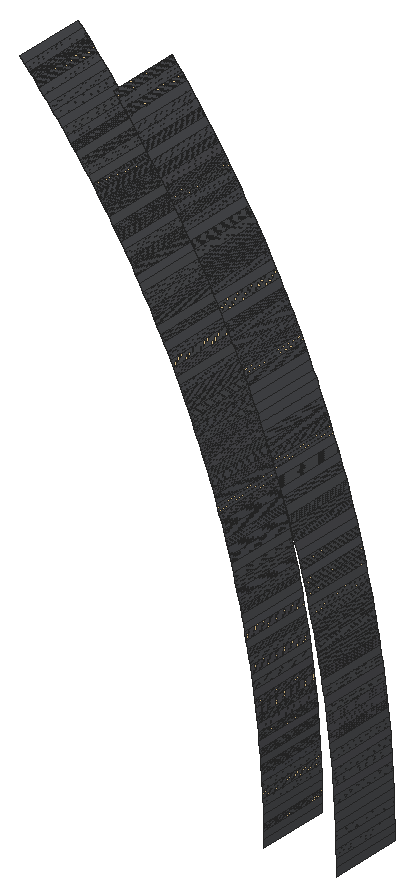
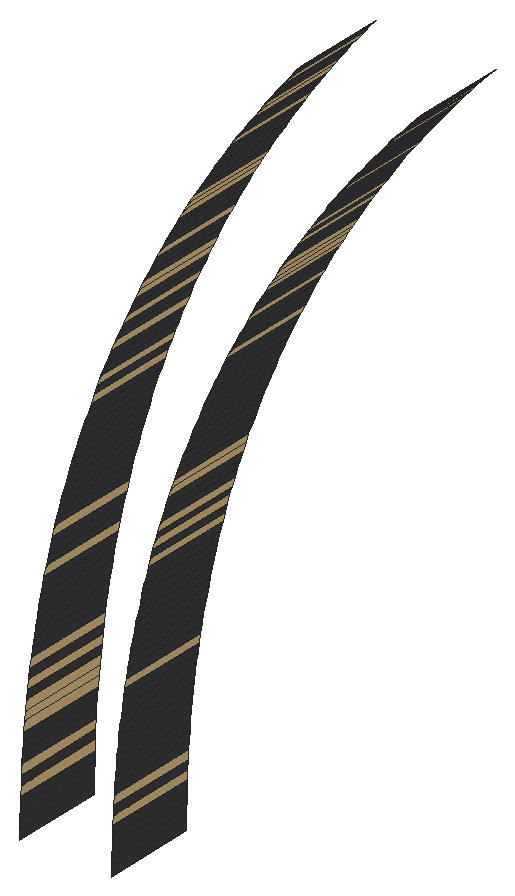
# SketchUp Ruby script. Lengths in inches.
U = 1.inch
M = Sketchup.active_model
def pt(a) = Geom::Point3d.new(a.map { |v| v * U })
def face(e, loops, mat)
  f = e.add_face(loops[0].map { |a| pt(a) })
  loops[1..].each { |l| e.add_face(l.map { |a| pt(a) }).erase! }
  f.material = f.back_material = mat if mat
  f
end
# faces: each face lists its corners as indices into pts; further lists are holes
def faces(e, pts, list, mat = nil) = list.each { |f| face(e, (f[0].is_a?(Array) ? f : [f]).map { |l| l.map { |i| pts[i] } }, mat) }
# xy, xz, yz: faces in a plane at the given z, y or x. An outline is a flat list of corners, or four numbers for a rectangle; further outlines are holes
def ring(l) = l.size == 4 ? [[l[0], l[1]], [l[2], l[1]], [l[2], l[3]], [l[0], l[3]]] : l.each_slice(2).to_a
def flat(e, list, mat, &to3) = list.each { |f| face(e, (f[0].is_a?(Array) ? f : [f]).map { |l| ring(l).map { |u, v| to3.(u, v) } }, mat) }
def xy(e, z, list, mat = nil) = flat(e, list, mat) { |x, y| [x, y, z] }
def xz(e, y, list, mat = nil) = flat(e, list, mat) { |x, z| [x, y, z] }
def yz(e, x, list, mat = nil) = flat(e, list, mat) { |y, z| [x, y, z] }
def lines(e, pts, list) = list.each { |a, b| e.add_line(pt(pts[a]), pt(pts[b])) }
# prism: a flat outline (further loops are holes) pulled along v
def prism(e, loops, v, mat = nil)
  f = face(e, loops, mat); d = Geom::Vector3d.new(v.map { |x| x * U })
  f.pushpull(f.normal.samedirection?(d) ? d.length : -d.length)
end
def box(e, o, s, mat = nil) = prism(e, [[o, [o[0] + s[0], o[1], o[2]], [o[0] + s[0], o[1] + s[1], o[2]], [o[0], o[1] + s[1], o[2]]]], [0, 0, s[2]], mat)
def at(x, y, z, deg = 0) = Geom::Transformation.translation(pt([x, y, z])) * Geom::Transformation.rotation(ORIGIN, Z_AXIS, deg.degrees)
def axes(o, x, y, z) = Geom::Transformation.new([*x, 0, *y, 0, *z, 0, *pt(o).to_a, 1])
def part(name) = M.definitions.add(name)
# library, detail: a bought-in or finely detailed component or shape, given as its bounding box
def library(name, o, s) = part(name).tap { |d| box(d.entities, o, s) }
def detail(e, o, s) = box(e.add_group.entities, o, s)
def put(e, d, t, mat = nil) = e.add_instance(d, t).tap { |i| i.material = mat if mat }
def group(e, t, mat = nil) = e.add_group.tap { |g| g.transformation = t; g.material = mat if mat }.entities
root = M.entities
M.materials.add("1432 AP 8245 TAR ROAD").color = [71, 72, 75]
M.materials.add("Outer Light").color = [251, 217, 152]
yz(root,555.99,[[95.37,561.24,96.87,561.39],[95.37,561.39,96.87,561.54]],"1432 AP 8245 TAR ROAD")
yz(root,555.99,[[95.37,561.24,96.87,561.39],[95.37,561.39,96.87,561.54]],"Outer Light")
yz(root,556,[[95.37,560.79,96.87,560.94],[95.37,560.94,96.87,561.09]],"1432 AP 8245 TAR ROAD")
yz(root,556,[[95.37,560.79,96.87,560.94],[95.37,560.94,96.87,561.09]],"Outer Light")
yz(root,557.48,[[95.37,561.6,96.87,561.76]],"1432 AP 8245 TAR ROAD")
yz(root,557.48,[[95.37,561.6,96.87,561.76]],"Outer Light")
yz(root,557.49,[[95.37,561.28,96.87,561.4375]],"1432 AP 8245 TAR ROAD")
yz(root,557.49,[[95.37,561.28,96.87,561.4375]],"Outer Light")
yz(root,557.5,[[95.37,560.79,96.87,560.95],[95.37,560.95,96.87,561.11]],"1432 AP 8245 TAR ROAD")
yz(root,557.5,[[95.37,560.79,96.87,560.95],[95.37,560.95,96.87,561.11]],"Outer Light")
p = [[555.99,95.37,561.24],[556,95.37,561.09],[556,96.87,561.09],[555.99,96.87,561.24],[555.99,96.87,561.24],[556,96.87,561.09],
  [556,95.37,561.09],[555.99,95.37,561.24],[557.5,95.37,561.11],[557.49,95.37,561.28],[557.49,96.87,561.28],[557.5,96.87,561.11],
  [557.5,96.87,561.11],[557.49,96.87,561.28],[557.49,95.37,561.28],[557.5,95.37,561.11],[557.49,95.37,561.4375],[557.48,95.37,561.6],
  [557.48,96.87,561.6],[557.49,96.87,561.4375],[557.49,96.87,561.4375],[557.48,96.87,561.6],[557.48,95.37,561.6],[557.49,95.37,561.4375],
  [555.98,95.37,561.6875],[555.99,95.37,561.54],[555.99,96.87,561.54],[555.98,96.87,561.6875],[555.98,96.87,561.6875],[555.99,96.87,561.54],
  [555.99,95.37,561.54],[555.98,95.37,561.6875],[555.97,95.37,561.84],[555.97,96.87,561.84],[555.97,96.87,561.84],[555.97,95.37,561.84],
  [555.96,95.37,561.99],[555.96,96.87,561.99],[555.96,96.87,561.99],[555.96,95.37,561.99],[557.48,95.37,561.76],[557.47,95.37,561.92],
  [557.47,96.87,561.92],[557.48,96.87,561.76],[557.48,96.87,561.76],[557.47,96.87,561.92],[557.47,95.37,561.92],[557.48,95.37,561.76],
  [557.46,95.37,562.08],[557.46,96.87,562.08],[557.46,96.87,562.08],[557.46,95.37,562.08],[555.95,95.37,562.13],[555.95,96.87,562.13],
  [555.95,96.87,562.13],[555.95,95.37,562.13],[555.94,95.37,562.28],[555.94,96.87,562.28],[555.94,96.87,562.28],[555.94,95.37,562.28],
  [557.45,95.37,562.24],[557.45,96.87,562.24],[557.45,96.87,562.24],[557.45,95.37,562.24],[557.4375,95.37,562.4],[557.4375,96.87,562.4],
  [557.4375,96.87,562.4],[557.4375,95.37,562.4],[555.93,95.37,562.43],[555.93,96.87,562.43],[555.93,96.87,562.43],[555.93,95.37,562.43],
  [555.92,95.37,562.58],[555.92,96.87,562.58],[555.92,96.87,562.58],[555.92,95.37,562.58],[557.42,95.37,562.5625],[557.42,96.87,562.5625],
  [557.42,96.87,562.5625],[557.42,95.37,562.5625],[555.9,95.37,562.73],[555.9,96.87,562.73],[555.9,96.87,562.73],[555.9,95.37,562.73],
  [557.41,95.37,562.72],[557.41,96.87,562.72],[557.41,96.87,562.72],[557.41,95.37,562.72],[555.89,95.37,562.88],[555.89,96.87,562.88],
  [555.89,96.87,562.88],[555.89,95.37,562.88],[557.39,95.37,562.88],[557.39,96.87,562.88],[557.39,96.87,562.88],[557.39,95.37,562.88],
  [555.87,95.37,563.03],[555.87,96.87,563.03],[555.87,96.87,563.03],[555.87,95.37,563.03],[557.375,95.37,563.04],[557.375,96.87,563.04],
  [557.375,96.87,563.04],[557.375,95.37,563.04],[555.85,95.37,563.17],[555.85,96.87,563.17],[555.85,96.87,563.17],[555.85,95.37,563.17],
  [557.36,95.37,563.2],[557.36,96.87,563.2],[557.36,96.87,563.2],[557.36,95.37,563.2],[555.83,95.37,563.32],[555.83,96.87,563.32],
  [555.83,96.87,563.32],[555.83,95.37,563.32],[557.34,95.37,563.36],[557.34,96.87,563.36],[557.34,96.87,563.36],[557.34,95.37,563.36],
  [555.81,95.37,563.47],[555.81,96.87,563.47],[555.81,96.87,563.47],[555.81,95.37,563.47],[557.32,95.37,563.52],[557.32,96.87,563.52],
  [557.32,96.87,563.52],[557.32,95.37,563.52],[555.79,95.37,563.62],[555.79,96.87,563.62],[555.79,96.87,563.62],[555.79,95.37,563.62],
  [557.3,95.37,563.68],[557.3,96.87,563.68],[557.3,96.87,563.68],[557.3,95.37,563.68],[555.77,95.37,563.76],[555.77,96.87,563.76],
  [555.77,96.87,563.76],[555.77,95.37,563.76],[557.27,95.37,563.84],[557.27,96.87,563.84],[557.27,96.87,563.84],[557.27,95.37,563.84],
  [555.74,95.37,563.91],[555.74,96.87,563.91],[555.74,96.87,563.91],[555.74,95.37,563.91],[557.25,95.37,564],[557.25,96.87,564],
  [557.25,96.87,564],[557.25,95.37,564],[555.72,95.37,564.06],[555.72,96.87,564.06],[555.72,96.87,564.06],[555.72,95.37,564.06],
  [557.22,95.37,564.16],[557.22,96.87,564.16],[557.22,96.87,564.16],[557.22,95.37,564.16],[555.69,95.37,564.21],[555.69,96.87,564.21],
  [555.69,96.87,564.21],[555.69,95.37,564.21],[555.66,95.37,564.35],[555.66,96.87,564.35],[555.66,96.87,564.35],[555.66,95.37,564.35],
  [557.19,95.37,564.32],[557.19,96.87,564.32],[557.19,96.87,564.32],[557.19,95.37,564.32],[557.17,95.37,564.48],[557.17,96.87,564.48],
  [557.17,96.87,564.48],[557.17,95.37,564.48],[555.63,95.37,564.5],[555.63,96.87,564.5],[555.63,96.87,564.5],[555.63,95.37,564.5],
  [555.61,95.37,564.65],[555.61,96.87,564.65],[555.61,96.87,564.65],[555.61,95.37,564.65],[557.14,95.37,564.63],[557.14,96.87,564.63],
  [557.14,96.87,564.63],[557.14,95.37,564.63],[555.57,95.37,564.79],[555.57,96.87,564.79],[555.57,96.87,564.79],[555.57,95.37,564.79],
  [557.11,95.37,564.79],[557.11,96.87,564.79],[557.11,96.87,564.79],[557.11,95.37,564.79],[555.54,95.37,564.9375],[555.54,96.87,564.9375],
  [555.54,96.87,564.9375],[555.54,95.37,564.9375],[557.07,95.37,564.95],[557.07,96.87,564.95],[557.07,96.87,564.95],[557.07,95.37,564.95],
  [555.51,95.37,565.08],[555.51,96.87,565.08],[555.51,96.87,565.08],[555.51,95.37,565.08],[557.04,95.37,565.11],[557.04,96.87,565.11],
  [557.04,96.87,565.11],[557.04,95.37,565.11],[555.48,95.37,565.23],[555.48,96.87,565.23],[555.48,96.87,565.23],[555.48,95.37,565.23],
  [557.01,95.37,565.26],[557.01,96.87,565.26],[557.01,96.87,565.26],[557.01,95.37,565.26],[555.44,95.37,565.37],[555.44,96.87,565.37],
  [555.44,96.87,565.37],[555.44,95.37,565.37],[556.97,95.37,565.42],[556.97,96.87,565.42],[556.97,96.87,565.42],[556.97,95.37,565.42],
  [555.4,95.37,565.52],[555.4,96.87,565.52],[555.4,96.87,565.52],[555.4,95.37,565.52],[556.93,95.37,565.58],[556.93,96.87,565.58],
  [556.93,96.87,565.58],[556.93,95.37,565.58],[555.37,95.37,565.66],[555.37,96.87,565.66],[555.37,96.87,565.66],[555.37,95.37,565.66],
  [556.9,95.37,565.73],[556.9,96.87,565.73],[556.9,96.87,565.73],[556.9,95.37,565.73],[555.33,95.37,565.81],[555.33,96.87,565.81],
  [555.33,96.87,565.81],[555.33,95.37,565.81],[556.86,95.37,565.89],[556.86,96.87,565.89],[556.86,96.87,565.89],[556.86,95.37,565.89],
  [555.29,95.37,565.95],[555.29,96.87,565.95],[555.29,96.87,565.95],[555.29,95.37,565.95],[555.25,95.37,566.09],[555.25,96.87,566.09],
  [555.25,96.87,566.09],[555.25,95.37,566.09],[556.82,95.37,566.05],[556.82,96.87,566.05],[556.82,96.87,566.05],[556.82,95.37,566.05],
  [556.77,95.37,566.2],[556.77,96.87,566.2],[556.77,96.87,566.2],[556.77,95.37,566.2],[555.2,95.37,566.24],[555.2,96.87,566.24],
  [555.2,96.87,566.24],[555.2,95.37,566.24],[555.16,95.37,566.38],[555.16,96.87,566.38],[555.16,96.87,566.38],[555.16,95.37,566.38],
  [556.73,95.37,566.36],[556.73,96.87,566.36],[556.73,96.87,566.36],[556.73,95.37,566.36],[555.12,95.37,566.52],[555.12,96.87,566.52],
  [555.12,96.87,566.52],[555.12,95.37,566.52],[556.6875,95.37,566.51],[556.6875,96.87,566.51],[556.6875,96.87,566.51],[556.6875,95.37,566.51],
  [555.07,95.37,566.66],[555.07,96.87,566.66],[555.07,96.87,566.66],[555.07,95.37,566.66],[556.64,95.37,566.67],[556.64,96.87,566.67],
  [556.64,96.87,566.67],[556.64,95.37,566.67],[555.02,95.37,566.81],[555.02,96.87,566.81],[555.02,96.87,566.81],[555.02,95.37,566.81],
  [556.59,95.37,566.82],[556.59,96.87,566.82],[556.59,96.87,566.82],[556.59,95.37,566.82],[554.98,95.37,566.95],[554.98,96.87,566.95],
  [554.98,96.87,566.95],[554.98,95.37,566.95],[556.55,95.37,566.97],[556.55,96.87,566.97],[556.55,96.87,566.97],[556.55,95.37,566.97],
  [554.93,95.37,567.09],[554.93,96.87,567.09],[554.93,96.87,567.09],[554.93,95.37,567.09],[556.5,95.37,567.125],[556.5,96.87,567.125],
  [556.5,96.87,567.125],[556.5,95.37,567.125],[554.875,95.37,567.23],[554.875,96.87,567.23],[554.875,96.87,567.23],[554.875,95.37,567.23],
  [556.45,95.37,567.28],[556.45,96.87,567.28],[556.45,96.87,567.28],[556.45,95.37,567.28],[554.83,95.37,567.37],[554.83,96.87,567.37],
  [554.83,96.87,567.37],[554.83,95.37,567.37],[556.39,95.37,567.43],[556.39,96.87,567.43],[556.39,96.87,567.43],[556.39,95.37,567.43],
  [554.77,95.37,567.51],[554.77,96.87,567.51],[554.77,96.87,567.51],[554.77,95.37,567.51],[556.34,95.37,567.58],[556.34,96.87,567.58],
  [556.34,96.87,567.58],[556.34,95.37,567.58],[554.72,95.37,567.65],[554.72,96.87,567.65],[554.72,96.87,567.65],[554.72,95.37,567.65],
  [554.67,95.37,567.79],[554.67,96.87,567.79],[554.67,96.87,567.79],[554.67,95.37,567.79],[556.29,95.37,567.74],[556.29,96.87,567.74],
  [556.29,96.87,567.74],[556.29,95.37,567.74],[556.23,95.37,567.89],[556.23,96.87,567.89],[556.23,96.87,567.89],[556.23,95.37,567.89],
  [554.61,95.37,567.92],[554.61,96.87,567.92],[554.61,96.87,567.92],[554.61,95.37,567.92],[554.55,95.37,568.0625],[554.55,96.87,568.0625],
  [554.55,96.87,568.0625],[554.55,95.37,568.0625],[556.18,95.37,568.04],[556.18,96.87,568.04],[556.18,96.87,568.04],[556.18,95.37,568.04],
  [556.12,95.37,568.1875],[556.12,96.87,568.1875],[556.12,96.87,568.1875],[556.12,95.37,568.1875],[554.5,95.37,568.2],[554.5,96.87,568.2],
  [554.5,96.87,568.2],[554.5,95.37,568.2],[554.4375,95.37,568.34],[554.4375,96.87,568.34],[554.4375,96.87,568.34],[554.4375,95.37,568.34],
  [556.06,95.37,568.34],[556.06,96.87,568.34],[556.06,96.87,568.34],[556.06,95.37,568.34],[554.38,95.37,568.47],[554.38,96.87,568.47],
  [554.38,96.87,568.47],[554.38,95.37,568.47],[556,95.37,568.49],[556,96.87,568.49],[556,96.87,568.49],[556,95.37,568.49],
  [554.32,95.37,568.61],[554.32,96.87,568.61],[554.32,96.87,568.61],[554.32,95.37,568.61],[555.94,95.37,568.64],[555.94,96.87,568.64],
  [555.94,96.87,568.64],[555.94,95.37,568.64],[554.25,95.37,568.75],[554.25,96.87,568.75],[554.25,96.87,568.75],[554.25,95.37,568.75],
  [555.88,95.37,568.79],[555.88,96.87,568.79],[555.88,96.87,568.79],[555.88,95.37,568.79],[554.19,95.37,568.88],[554.19,96.87,568.88],
  [554.19,96.87,568.88],[554.19,95.37,568.88],[555.8125,95.37,568.93],[555.8125,96.87,568.93],[555.8125,96.87,568.93],[555.8125,95.37,568.93],
  [554.13,95.37,569.02],[554.13,96.87,569.02],[554.13,96.87,569.02],[554.13,95.37,569.02],[555.75,95.37,569.08],[555.75,96.87,569.08],
  [555.75,96.87,569.08],[555.75,95.37,569.08],[554.0625,95.37,569.15],[554.0625,96.87,569.15],[554.0625,96.87,569.15],[554.0625,95.37,569.15],
  [555.68,95.37,569.23],[555.68,96.87,569.23],[555.68,96.87,569.23],[555.68,95.37,569.23],[554,95.37,569.28],[554,96.87,569.28],
  [554,96.87,569.28],[554,95.37,569.28],[555.62,95.37,569.375],[555.62,96.87,569.375],[555.62,96.87,569.375],[555.62,95.37,569.375],
  [553.93,95.37,569.42],[553.93,96.87,569.42],[553.93,96.87,569.42],[553.93,95.37,569.42],[553.86,95.37,569.55],[553.86,96.87,569.55],
  [553.86,96.87,569.55],[553.86,95.37,569.55],[555.55,95.37,569.52],[555.55,96.87,569.52],[555.55,96.87,569.52],[555.55,95.37,569.52],
  [555.48,95.37,569.67],[555.48,96.87,569.67],[555.48,96.87,569.67],[555.48,95.37,569.67],[553.79,95.37,569.68],[553.79,96.87,569.68],
  [553.79,96.87,569.68],[553.79,95.37,569.68],[553.72,95.37,569.8125],[553.72,96.87,569.8125],[553.72,96.87,569.8125],[553.72,95.37,569.8125],
  [555.41,95.37,569.8125],[555.41,96.87,569.8125],[555.41,96.87,569.8125],[555.41,95.37,569.8125],[553.65,95.37,569.95],[553.65,96.87,569.95],
  [553.65,96.87,569.95],[553.65,95.37,569.95],[555.34,95.37,569.96],[555.34,96.87,569.96],[555.34,96.87,569.96],[555.34,95.37,569.96],
  [553.58,95.37,570.08],[553.58,96.87,570.08],[553.58,96.87,570.08],[553.58,95.37,570.08],[555.27,95.37,570.1],[555.27,96.87,570.1],
  [555.27,96.87,570.1],[555.27,95.37,570.1],[553.5,95.37,570.21],[553.5,96.87,570.21],[553.5,96.87,570.21],[553.5,95.37,570.21],
  [555.19,95.37,570.24],[555.19,96.87,570.24],[555.19,96.87,570.24],[555.19,95.37,570.24],[553.43,95.37,570.34],[553.43,96.87,570.34],
  [553.43,96.87,570.34],[553.43,95.37,570.34],[555.12,95.37,570.38],[555.12,96.87,570.38],[555.12,96.87,570.38],[555.12,95.37,570.38],
  [553.35,95.37,570.46],[553.35,96.87,570.46],[553.35,96.87,570.46],[553.35,95.37,570.46],[555.04,95.37,570.53],[555.04,96.87,570.53],
  [555.04,96.87,570.53],[555.04,95.37,570.53],[553.28,95.37,570.59],[553.28,96.87,570.59],[553.28,96.87,570.59],[553.28,95.37,570.59],
  [554.96,95.37,570.67],[554.96,96.87,570.67],[554.96,96.87,570.67],[554.96,95.37,570.67],[553.2,95.37,570.72],[553.2,96.87,570.72],
  [553.2,96.87,570.72],[553.2,95.37,570.72],[553.12,95.37,570.85],[553.12,96.87,570.85],[553.12,96.87,570.85],[553.12,95.37,570.85],
  [554.89,95.37,570.81],[554.89,96.87,570.81],[554.89,96.87,570.81],[554.89,95.37,570.81],[553.04,95.37,570.97],[553.04,96.87,570.97],
  [553.04,96.87,570.97],[553.04,95.37,570.97],[554.81,95.37,570.95],[554.81,96.87,570.95],[554.81,96.87,570.95],[554.81,95.37,570.95],
  [554.73,95.37,571.09],[554.73,96.87,571.09],[554.73,96.87,571.09],[554.73,95.37,571.09],[552.96,95.37,571.1],[552.96,96.87,571.1],
  [552.96,96.87,571.1],[552.96,95.37,571.1],[552.88,95.37,571.22],[552.88,96.87,571.22],[552.88,96.87,571.22],[552.88,95.37,571.22],
  [554.65,95.37,571.23],[554.65,96.87,571.23],[554.65,96.87,571.23],[554.65,95.37,571.23],[552.8,95.37,571.35],[552.8,96.87,571.35],
  [552.8,96.87,571.35],[552.8,95.37,571.35],[554.5625,95.37,571.37],[554.5625,96.87,571.37],[554.5625,96.87,571.37],[554.5625,95.37,571.37],
  [552.71,95.37,571.47],[552.71,96.87,571.47],[552.71,96.87,571.47],[552.71,95.37,571.47],[554.48,95.37,571.5],[554.48,96.87,571.5],
  [554.48,96.87,571.5],[554.48,95.37,571.5],[552.63,95.37,571.59],[552.63,96.87,571.59],[552.63,96.87,571.59],[552.63,95.37,571.59],
  [554.39,95.37,571.64],[554.39,96.87,571.64],[554.39,96.87,571.64],[554.39,95.37,571.64],[552.54,95.37,571.72],[552.54,96.87,571.72],
  [552.54,96.87,571.72],[552.54,95.37,571.72],[554.31,95.37,571.78],[554.31,96.87,571.78],[554.31,96.87,571.78],[554.31,95.37,571.78],
  [552.46,95.37,571.84],[552.46,96.87,571.84],[552.46,96.87,571.84],[552.46,95.37,571.84],[552.37,95.37,571.96],[552.37,96.87,571.96],
  [552.37,96.87,571.96],[552.37,95.37,571.96],[554.22,95.37,571.91],[554.22,96.87,571.91],[554.22,96.87,571.91],[554.22,95.37,571.91],
  [554.13,95.37,572.05],[554.13,96.87,572.05],[554.13,96.87,572.05],[554.13,95.37,572.05],[552.28,95.37,572.08],[552.28,96.87,572.08],
  [552.28,96.87,572.08],[552.28,95.37,572.08],[554.05,95.37,572.18],[554.05,96.87,572.18],[554.05,96.87,572.18],[554.05,95.37,572.18],
  [552.19,95.37,572.2],[552.19,96.87,572.2],[552.19,96.87,572.2],[552.19,95.37,572.2],[552.1,95.37,572.32],[552.1,96.87,572.32],
  [552.1,96.87,572.32],[552.1,95.37,572.32],[553.96,95.37,572.31],[553.96,96.87,572.31],[553.96,96.87,572.31],[553.96,95.37,572.31],
  [552.01,95.37,572.4375],[552.01,96.87,572.4375],[552.01,96.87,572.4375],[552.01,95.37,572.4375],[553.86,95.37,572.45],[553.86,96.87,572.45],
  [553.86,96.87,572.45],[553.86,95.37,572.45],[551.92,95.37,572.55],[551.92,96.87,572.55],[551.92,96.87,572.55],[551.92,95.37,572.55],
  [553.77,95.37,572.58],[553.77,96.87,572.58],[553.77,96.87,572.58],[553.77,95.37,572.58],[551.83,95.37,572.67],[551.83,96.87,572.67],
  [551.83,96.87,572.67],[551.83,95.37,572.67],[553.68,95.37,572.71],[553.68,96.87,572.71],[553.68,96.87,572.71],[553.68,95.37,572.71],
  [551.73,95.37,572.79],[551.73,96.87,572.79],[551.73,96.87,572.79],[551.73,95.37,572.79],[553.58,95.37,572.84],[553.58,96.87,572.84],
  [553.58,96.87,572.84],[553.58,95.37,572.84],[551.64,95.37,572.9],[551.64,96.87,572.9],[551.64,96.87,572.9],[551.64,95.37,572.9],
  [553.49,95.37,572.97],[553.49,96.87,572.97],[553.49,96.87,572.97],[553.49,95.37,572.97],[551.54,95.37,573.02],[551.54,96.87,573.02],
  [551.54,96.87,573.02],[551.54,95.37,573.02],[551.45,95.37,573.13],[551.45,96.87,573.13],[551.45,96.87,573.13],[551.45,95.37,573.13],
  [553.39,95.37,573.1],[553.39,96.87,573.1],[553.39,96.87,573.1],[553.39,95.37,573.1],[551.35,95.37,573.24],[551.35,96.87,573.24],
  [551.35,96.87,573.24],[551.35,95.37,573.24],[553.3,95.37,573.23],[553.3,96.87,573.23],[553.3,96.87,573.23],[553.3,95.37,573.23],
  [551.25,95.37,573.36],[551.25,96.87,573.36],[551.25,96.87,573.36],[551.25,95.37,573.36],[553.2,95.37,573.36],[553.2,96.87,573.36],
  [553.2,96.87,573.36],[553.2,95.37,573.36],[551.15,95.37,573.47],[551.15,96.87,573.47],[551.15,96.87,573.47],[551.15,95.37,573.47],
  [553.1,95.37,573.48],[553.1,96.87,573.48],[553.1,96.87,573.48],[553.1,95.37,573.48],[551.05,95.37,573.58],[551.05,96.87,573.58],
  [551.05,96.87,573.58],[551.05,95.37,573.58],[553,95.37,573.61],[553,96.87,573.61],[553,96.87,573.61],[553,95.37,573.61],
  [550.95,95.37,573.6875],[550.95,96.87,573.6875],[550.95,96.87,573.6875],[550.95,95.37,573.6875],[552.9,95.37,573.73],[552.9,96.87,573.73],
  [552.9,96.87,573.73],[552.9,95.37,573.73]]
faces(root,p,[[0,1,2,3],[8,9,10,11],[16,17,18,19],[24,25,26,27],[32,24,27,33],[36,32,33,37],[40,41,42,43],[41,48,49,42],
  [52,36,37,53],[56,52,53,57],[48,60,61,49],[60,64,65,61],[68,56,57,69],[72,68,69,73],[64,76,77,65],[80,72,73,81],
  [76,84,85,77],[88,80,81,89],[84,92,93,85],[96,88,89,97],[92,100,101,93],[104,96,97,105],[100,108,109,101],[112,104,105,113],
  [108,116,117,109],[120,112,113,121],[116,124,125,117],[128,120,121,129],[124,132,133,125],[136,128,129,137],[132,140,141,133],[144,136,137,145],
  [140,148,149,141],[152,144,145,153],[148,156,157,149],[160,152,153,161],[164,160,161,165],[156,168,169,157],[168,172,173,169],[176,164,165,177],
  [180,176,177,181],[172,184,185,173],[188,180,181,189],[184,192,193,185],[196,188,189,197],[192,200,201,193],[204,196,197,205],[200,208,209,201],
  [212,204,205,213],[208,216,217,209],[220,212,213,221],[216,224,225,217],[228,220,221,229],[224,232,233,225],[236,228,229,237],[232,240,241,233],
  [244,236,237,245],[240,248,249,241],[252,244,245,253],[256,252,253,257],[248,260,261,249],[260,264,265,261],[268,256,257,269],[272,268,269,273],
  [264,276,277,265],[280,272,273,281],[276,284,285,277],[288,280,281,289],[284,292,293,285],[296,288,289,297],[292,300,301,293],[304,296,297,305],
  [300,308,309,301],[312,304,305,313],[308,316,317,309],[320,312,313,321],[316,324,325,317],[328,320,321,329],[324,332,333,325],[336,328,329,337],
  [332,340,341,333],[344,336,337,345],[348,344,345,349],[340,352,353,341],[352,356,357,353],[360,348,349,361],[364,360,361,365],[356,368,369,357],
  [368,372,373,369],[376,364,365,377],[380,376,377,381],[372,384,385,373],[388,380,381,389],[384,392,393,385],[396,388,389,397],[392,400,401,393],
  [404,396,397,405],[400,408,409,401],[412,404,405,413],[408,416,417,409],[420,412,413,421],[416,424,425,417],[428,420,421,429],[424,432,433,425],
  [436,428,429,437],[432,440,441,433],[444,436,437,445],[448,444,445,449],[440,452,453,441],[452,456,457,453],[460,448,449,461],[464,460,461,465],
  [456,468,469,457],[472,464,465,473],[468,476,477,469],[480,472,473,481],[476,484,485,477],[488,480,481,489],[484,492,493,485],[496,488,489,497],
  [492,500,501,493],[504,496,497,505],[500,508,509,501],[512,504,505,513],[508,516,517,509],[520,512,513,521],[524,520,521,525],[516,528,529,517],
  [532,524,525,533],[528,536,537,529],[536,540,541,537],[544,532,533,545],[548,544,545,549],[540,552,553,541],[556,548,549,557],[552,560,561,553],
  [564,556,557,565],[560,568,569,561],[572,564,565,573],[568,576,577,569],[580,572,573,581],[576,584,585,577],[588,580,581,589],[592,588,589,593],
  [584,596,597,585],[596,600,601,597],[604,592,593,605],[600,608,609,601],[612,604,605,613],[616,612,613,617],[608,620,621,609],[624,616,617,625],
  [620,628,629,621],[632,624,625,633],[628,636,637,629],[640,632,633,641],[636,644,645,637],[648,640,641,649],[644,652,653,645],[656,648,649,657],
  [652,660,661,653],[664,656,657,665],[668,664,665,669],[660,672,673,661],[676,668,669,677],[672,680,681,673],[684,676,677,685],[680,688,689,681],
  [692,684,685,693],[688,696,697,689],[700,692,693,701],[696,704,705,697],[708,700,701,709],[704,712,713,705]],"1432 AP 8245 TAR ROAD")
faces(root,p,[[4,5,6,7],[12,13,14,15],[20,21,22,23],[28,29,30,31],[34,28,31,35],[38,34,35,39],[44,45,46,47],[45,50,51,46],
  [54,38,39,55],[58,54,55,59],[50,62,63,51],[62,66,67,63],[70,58,59,71],[74,70,71,75],[66,78,79,67],[82,74,75,83],
  [78,86,87,79],[90,82,83,91],[86,94,95,87],[98,90,91,99],[94,102,103,95],[106,98,99,107],[102,110,111,103],[114,106,107,115],
  [110,118,119,111],[122,114,115,123],[118,126,127,119],[130,122,123,131],[126,134,135,127],[138,130,131,139],[134,142,143,135],[146,138,139,147],
  [142,150,151,143],[154,146,147,155],[150,158,159,151],[162,154,155,163],[166,162,163,167],[158,170,171,159],[170,174,175,171],[178,166,167,179],
  [182,178,179,183],[174,186,187,175],[190,182,183,191],[186,194,195,187],[198,190,191,199],[194,202,203,195],[206,198,199,207],[202,210,211,203],
  [214,206,207,215],[210,218,219,211],[222,214,215,223],[218,226,227,219],[230,222,223,231],[226,234,235,227],[238,230,231,239],[234,242,243,235],
  [246,238,239,247],[242,250,251,243],[254,246,247,255],[258,254,255,259],[250,262,263,251],[262,266,267,263],[270,258,259,271],[274,270,271,275],
  [266,278,279,267],[282,274,275,283],[278,286,287,279],[290,282,283,291],[286,294,295,287],[298,290,291,299],[294,302,303,295],[306,298,299,307],
  [302,310,311,303],[314,306,307,315],[310,318,319,311],[322,314,315,323],[318,326,327,319],[330,322,323,331],[326,334,335,327],[338,330,331,339],
  [334,342,343,335],[346,338,339,347],[350,346,347,351],[342,354,355,343],[354,358,359,355],[362,350,351,363],[366,362,363,367],[358,370,371,359],
  [370,374,375,371],[378,366,367,379],[382,378,379,383],[374,386,387,375],[390,382,383,391],[386,394,395,387],[398,390,391,399],[394,402,403,395],
  [406,398,399,407],[402,410,411,403],[414,406,407,415],[410,418,419,411],[422,414,415,423],[418,426,427,419],[430,422,423,431],[426,434,435,427],
  [438,430,431,439],[434,442,443,435],[446,438,439,447],[450,446,447,451],[442,454,455,443],[454,458,459,455],[462,450,451,463],[466,462,463,467],
  [458,470,471,459],[474,466,467,475],[470,478,479,471],[482,474,475,483],[478,486,487,479],[490,482,483,491],[486,494,495,487],[498,490,491,499],
  [494,502,503,495],[506,498,499,507],[502,510,511,503],[514,506,507,515],[510,518,519,511],[522,514,515,523],[526,522,523,527],[518,530,531,519],
  [534,526,527,535],[530,538,539,531],[538,542,543,539],[546,534,535,547],[550,546,547,551],[542,554,555,543],[558,550,551,559],[554,562,563,555],
  [566,558,559,567],[562,570,571,563],[574,566,567,575],[570,578,579,571],[582,574,575,583],[578,586,587,579],[590,582,583,591],[594,590,591,595],
  [586,598,599,587],[598,602,603,599],[606,594,595,607],[602,610,611,603],[614,606,607,615],[618,614,615,619],[610,622,623,611],[626,618,619,627],
  [622,630,631,623],[634,626,627,635],[630,638,639,631],[642,634,635,643],[638,646,647,639],[650,642,643,651],[646,654,655,647],[658,650,651,659],
  [654,662,663,655],[666,658,659,667],[670,666,667,671],[662,674,675,663],[678,670,671,679],[674,682,683,675],[686,678,679,687],[682,690,691,683],
  [694,686,687,695],[690,698,699,691],[702,694,695,703],[698,706,707,699],[710,702,703,711],[706,714,715,707]],"Outer Light")
